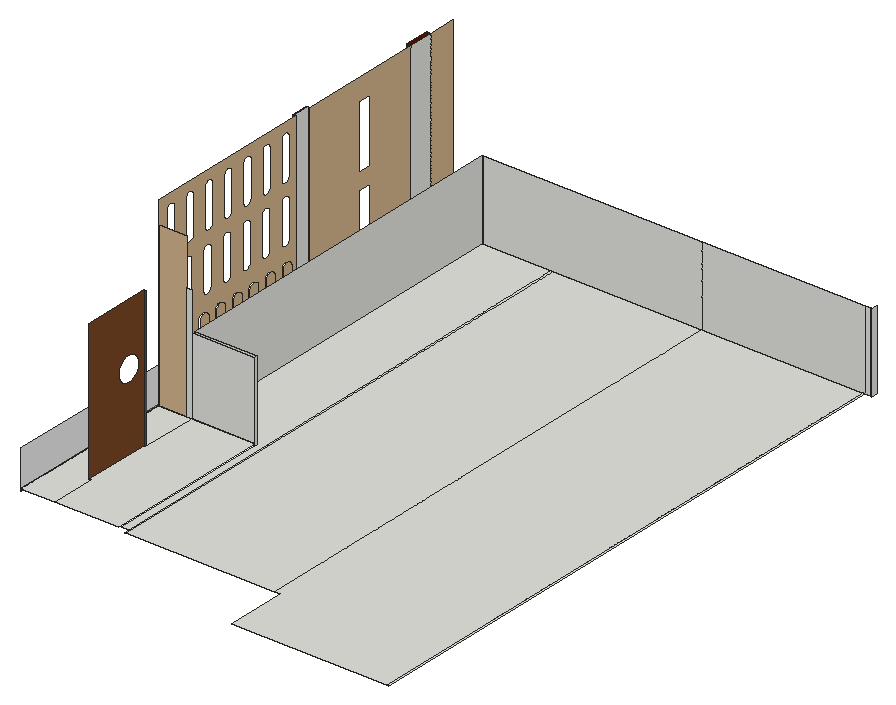
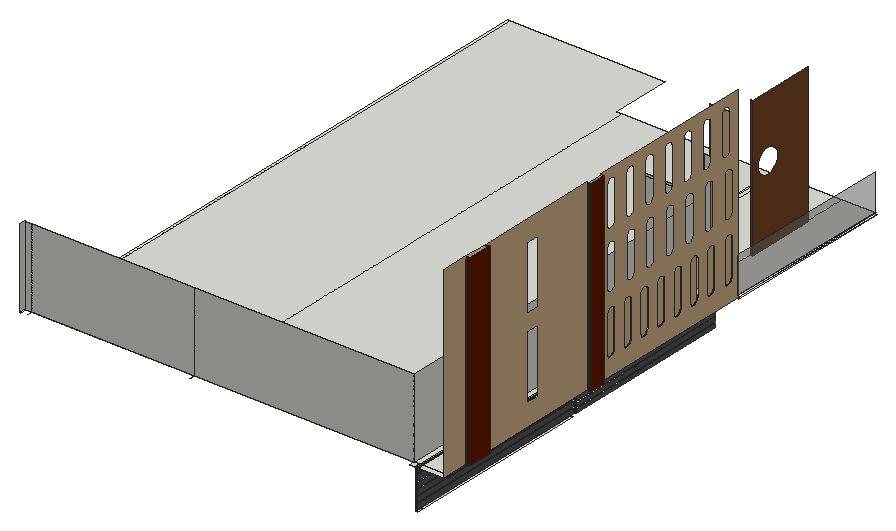
# SketchUp Ruby script. Lengths in inches.
U = 1.inch
M = Sketchup.active_model
def pt(a) = Geom::Point3d.new(a.map { |v| v * U })
def face(e, loops, mat)
  f = e.add_face(loops[0].map { |a| pt(a) })
  loops[1..].each { |l| e.add_face(l.map { |a| pt(a) }).erase! }
  f.material = f.back_material = mat if mat
  f
end
# faces: each face lists its corners as indices into pts; further lists are holes
def faces(e, pts, list, mat = nil) = list.each { |f| face(e, (f[0].is_a?(Array) ? f : [f]).map { |l| l.map { |i| pts[i] } }, mat) }
# xy, xz, yz: faces in a plane at the given z, y or x. An outline is a flat list of corners, or four numbers for a rectangle; further outlines are holes
def ring(l) = l.size == 4 ? [[l[0], l[1]], [l[2], l[1]], [l[2], l[3]], [l[0], l[3]]] : l.each_slice(2).to_a
def flat(e, list, mat, &to3) = list.each { |f| face(e, (f[0].is_a?(Array) ? f : [f]).map { |l| ring(l).map { |u, v| to3.(u, v) } }, mat) }
def xy(e, z, list, mat = nil) = flat(e, list, mat) { |x, y| [x, y, z] }
def xz(e, y, list, mat = nil) = flat(e, list, mat) { |x, z| [x, y, z] }
def yz(e, x, list, mat = nil) = flat(e, list, mat) { |y, z| [x, y, z] }
def lines(e, pts, list) = list.each { |a, b| e.add_line(pt(pts[a]), pt(pts[b])) }
# prism: a flat outline (further loops are holes) pulled along v
def prism(e, loops, v, mat = nil)
  f = face(e, loops, mat); d = Geom::Vector3d.new(v.map { |x| x * U })
  f.pushpull(f.normal.samedirection?(d) ? d.length : -d.length)
end
def box(e, o, s, mat = nil) = prism(e, [[o, [o[0] + s[0], o[1], o[2]], [o[0] + s[0], o[1] + s[1], o[2]], [o[0], o[1] + s[1], o[2]]]], [0, 0, s[2]], mat)
def at(x, y, z, deg = 0) = Geom::Transformation.translation(pt([x, y, z])) * Geom::Transformation.rotation(ORIGIN, Z_AXIS, deg.degrees)
def axes(o, x, y, z) = Geom::Transformation.new([*x, 0, *y, 0, *z, 0, *pt(o).to_a, 1])
def part(name) = M.definitions.add(name)
# library, detail: a bought-in or finely detailed component or shape, given as its bounding box
def library(name, o, s) = part(name).tap { |d| box(d.entities, o, s) }
def detail(e, o, s) = box(e.add_group.entities, o, s)
def put(e, d, t, mat = nil) = e.add_instance(d, t).tap { |i| i.material = mat if mat }
def group(e, t, mat = nil) = e.add_group.tap { |g| g.transformation = t; g.material = mat if mat }.entities
root = M.entities
M.materials.add("[0035_Tan]").color = [210, 180, 140]
M.materials.add("[Color B08]").color = [102, 25, 0]
M.materials.add("[Color M06]").color = [86, 86, 86]
M.materials.add("[Translucent Glass Gray]").color = [128, 128, 128]
M.materials["[Translucent Glass Gray]"].alpha = 0.5
M.materials.add("[Wood Veneer 01]").color = [120, 70, 37]
xy(root,120.75,[[90.83,1025.52,93.83,1311.7],[90.83,1311.7,93.83,1320.7]])
xy(root,122.27,[[90.83,755.01,93.83,1019.03]])
xy(root,123.5,[[90.83,1025.52,93.83,1320.7]])
xy(root,128.25,[[90.83,755.01,93.83,761.77],[90.83,761.77,93.83,1019.03]])
xy(root,130.625,[[90.83,1025.52,93.83,1311.7],[90.83,1311.7,93.83,1320.7]])
xy(root,130.89,[[90.83,755.01,93.83,1019.03]])
xy(root,133.375,[[90.83,1025.52,93.83,1320.7]])
xy(root,136.875,[[90.83,755.01,93.83,761.77],[90.83,761.77,93.83,1019.03]])
xy(root,139.52,[[90.83,755.01,93.83,1019.03]])
xy(root,140.5,[[90.83,1025.52,93.83,1311.7],[90.83,1311.7,93.83,1320.7]])
xy(root,143.25,[[90.83,1025.52,93.83,1320.7]])
xy(root,145.5,[[90.83,755.01,93.83,761.77],[90.83,761.77,93.83,1019.03]])
xy(root,148.14,[[90.83,755.01,93.83,1019.03]])
xy(root,150.375,[[90.83,1025.52,93.83,1311.7],[90.83,1311.7,93.83,1320.7]])
xy(root,153.125,[[90.83,1025.52,93.83,1320.7]])
xy(root,154.125,[[90.83,755.01,93.83,761.77],[90.83,761.77,93.83,1019.03]])
xy(root,156.77,[[90.83,755.01,93.83,1019.03]])
xy(root,160.25,[[90.83,1025.52,93.83,1311.7],[90.83,1311.7,93.83,1320.7]])
xy(root,162.75,[[90.83,755.01,93.83,761.77],[90.83,761.77,93.83,1019.03]])
xy(root,163,[[90.83,1025.52,93.83,1320.7]])
xy(root,165.39,[[90.83,755.01,93.83,1019.03]])
xy(root,170.125,[[90.83,1025.52,93.83,1311.7],[90.83,1311.7,93.83,1320.7]])
xy(root,171.375,[[90.83,755.01,93.83,761.77],[90.83,761.77,93.83,1019.03]])
xy(root,172.875,[[90.83,1025.52,93.83,1320.7]])
xy(root,174.02,[[90.83,755.01,93.83,1019.03]])
xy(root,180,[[446.36,406.51,446.36,499.93,437.36,499.93,437.36,1311.7,681.83,1311.7,681.83,406.51],[681.83,406.51,681.89,1311.7],[681.89,406.51,684.83,1311.7],[436.7,499.93,210.36,500.32,210.36,1311.7,436.7,1311.7],[436.7,499.93,437.36,1311.7],
  [208.04,500.32,210.36,1311.7],[49.08,501.15,49.08,761.77,51.64,761.77],[93.83,508.43,100.83,761.77],[100.83,508.43,102.83,761.77],[197.39,508.43,197.39,765.46,102.83,765.46,102.83,1311.7,208.04,1311.7,208.04,508.43],
  [90.83,755.01,93.83,761.77],[51.64,761.77,51.64,1022.51,48.64,1022.51,48.64,1047.49,51.64,1047.49,51.64,1311.7,90.83,1311.7,90.83,1025.52,87.83,1025.52,87.83,1019.03,90.83,1019.03,90.83,761.77],[93.83,761.77,93.83,1019.03,87.83,1019.03,87.83,1025.52,93.83,1025.52,93.83,1311.7,102.83,1311.7,102.83,761.77],[90.83,761.77,93.83,1019.03],[102.83,761.77,197.39,765.46],
  [102.83,761.77,197.39,765.46],[45.64,1022.51,48.64,1047.49],[90.83,1025.52,93.83,1311.7],[45.64,1240.86,51.64,1277.54],[51.64,1311.7,90.83,1320.7],
  [90.83,1311.7,93.83,1320.7],[93.83,1311.7,94.96,1320.7],[94.96,1311.7,102.83,1320.7],[693.83,1311.7,695.08,1320.7]])
xy(root,182.9375,[[49.08,502.77,49.1,502.77,51.64,761.77,49.08,761.77],[49.1,502.77,100.83,502.77,100.83,570.62,97.83,570.62,97.83,675.43,100.83,675.43,100.83,761.77,51.64,761.77],[100.83,502.77,197.39,502.77,197.39,761.77,100.83,761.77,100.83,675.43,97.83,675.43,97.83,570.62,100.83,570.62]])
xz(root,675.43,[[97.83,182.9375,100.83,394.5]],"[Wood Veneer 01]")
xz(root,755.01,[[90.83,122.27,93.83,128.25],[90.83,130.89,93.83,136.875],[90.83,139.52,93.83,145.5],[90.83,148.14,93.83,154.125],[90.83,156.77,93.83,162.75],
  [90.83,165.39,93.83,171.375],[90.83,174.02,93.83,180]])
xz(root,761.77,[[49.08,180,51.64,182.9375],[51.64,180,93.83,182.9375],[93.83,180,100.83,182.9375],[100.83,180,102.83,182.9375],[102.83,180,197.39,182.9375],
  [93.83,182.9375,100.83,358.375],[100.83,182.9375,197.39,300]])
xz(root,761.77,[[51.64,182.9375,93.83,429.125]],"[0035_Tan]")
xz(root,765.46,[[102.83,180,197.39,300]])
xz(root,1019.03,[[90.83,122.27,93.83,128.25],[90.83,130.89,93.83,136.875],[90.83,139.52,93.83,145.5],[90.83,148.14,93.83,154.125],[90.83,156.77,93.83,162.75],
  [90.83,165.39,93.83,171.375],[90.83,174.02,93.83,180]])
xz(root,1022.51,[[45.64,180,48.64,463.1875],[48.64,180,51.64,463.1875]],"[Color B08]")
xz(root,1025.52,[[90.83,123.5,93.83,130.625],[90.83,133.375,93.83,140.5],[90.83,143.25,93.83,150.375],[90.83,153.125,93.83,160.25],[90.83,163,93.83,170.125],
  [90.83,172.875,93.83,180]])
xz(root,1047.49,[[45.64,180,48.64,463.1875],[48.64,180,51.64,463.1875]],"[Color B08]")
xz(root,1240.86,[[45.64,180,51.64,463.1875]],"[Color B08]")
xz(root,1277.54,[[45.64,180,51.64,463.1875]],"[Color B08]")
xz(root,1311.7,[[102.83,180,103.71,300],[103.71,180,436.7,300],[436.7,180,684.83,300],[684.83,180,693.83,300],[693.83,180,695.08,300]])
xz(root,1320.7,[[90.83,123.5,93.83,130.625],[90.83,133.375,93.83,140.5],[90.83,143.25,93.83,150.375],[90.83,153.125,93.83,160.25],[90.83,163,93.83,170.125],
  [90.83,172.875,93.83,180]])
yz(root,45.64,[[1022.51,180,1047.49,463.1875],[1240.86,180,1277.54,463.1875]],"[Color B08]")
yz(root,48.64,[[1022.51,180,1047.49,463.1875]])
yz(root,51.64,[[1240.86,180,1277.54,463.1875]])
yz(root,51.64,[[[761.77,180,1022.51,463.1875],[1002.08,380.5625,1004.08,380.83,1005.94,381.6,1007.54,382.82,1008.77,384.42,1009.54,386.28,1009.8,388.28,1009.8,443.41,1009.2,445.06,1008.24,446.53,1006.99,447.77,1005.49,448.69,1003.83,449.27,1002.08,449.46,1000.33,449.27,998.67,448.69,997.18,447.77,995.92,446.53,994.97,445.06,994.36,443.41,994.36,388.28,994.625,386.28,995.4,384.42,996.625,382.82,998.22,381.6,1000.08,380.83],[965.71,380.5625,967.7,380.83,969.57,381.6,971.16,382.82,972.39,384.42,973.16,386.28,973.43,388.28,973.43,443.41,972.82,445.06,971.87,446.53,970.61,447.77,969.12,448.69,967.45,449.27,965.71,449.46,963.96,449.27,962.3,448.69,960.8,447.77,959.55,446.53,958.59,445.06,957.99,443.41,957.99,388.28,958.25,386.28,959.02,384.42,960.25,382.82,961.85,381.6,963.71,380.83],[929.33,380.5625,931.33,380.83,933.19,381.6,934.79,382.82,936.02,384.42,936.79,386.28,937.05,388.28,937.05,443.41,936.45,445.06,935.49,446.53,934.24,447.77,932.74,448.69,931.08,449.27,929.33,449.46,927.58,449.27,925.92,448.69,924.43,447.77,923.17,446.53,922.22,445.06,921.61,443.41,921.61,388.28,921.875,386.28,922.65,384.42,923.875,382.82,925.47,381.6,927.33,380.83],[892.96,380.5625,894.95,380.83,896.82,381.6,898.41,382.82,899.64,384.42,900.41,386.28,900.68,388.28,900.68,443.41,900.07,445.06,899.12,446.53,897.86,447.77,896.37,448.69,894.7,449.27,892.96,449.46,891.21,449.27,889.55,448.69,888.05,447.77,886.8,446.53,885.84,445.06,885.24,443.41,885.24,388.28,885.5,386.28,886.27,384.42,887.5,382.82,889.1,381.6,890.96,380.83],[856.58,380.5625,858.58,380.83,860.44,381.6,862.04,382.82,863.27,384.42,864.04,386.28,864.3,388.28,864.3,443.41,863.7,445.06,862.74,446.53,861.49,447.77,859.99,448.69,858.33,449.27,856.58,449.46,854.83,449.27,853.17,448.69,851.68,447.77,850.42,446.53,849.47,445.06,848.86,443.41,848.86,388.28,849.125,386.28,849.9,384.42,851.125,382.82,852.72,381.6,854.58,380.83],[820.21,380.5625,822.2,380.83,824.07,381.6,825.66,382.82,826.89,384.42,827.66,386.28,827.93,388.28,827.93,443.41,827.32,445.06,826.37,446.53,825.11,447.77,823.62,448.69,821.95,449.27,820.21,449.46,818.46,449.27,816.8,448.69,815.3,447.77,814.05,446.53,813.09,445.06,812.49,443.41,812.49,388.28,812.75,386.28,813.52,384.42,814.75,382.82,816.35,381.6,818.21,380.83],[783.83,380.5625,785.83,380.83,787.69,381.6,789.29,382.82,790.52,384.42,791.29,386.28,791.55,388.28,791.55,443.41,790.95,445.06,789.99,446.53,788.74,447.77,787.24,448.69,785.58,449.27,783.83,449.46,782.08,449.27,780.42,448.69,778.93,447.77,777.67,446.53,776.72,445.06,776.11,443.41,776.11,388.28,776.375,386.28,777.15,384.42,778.375,382.82,779.97,381.6,781.83,380.83],[1002.08,294.25,1004.08,294.51,1005.94,295.28,1007.54,296.51,1008.77,298.11,1009.54,299.97,1009.8,301.97,1009.8,357.09,1009.2,358.74,1008.24,360.22,1006.99,361.45,1005.49,362.38,1003.83,362.95,1002.08,363.15,1000.33,362.95,998.67,362.38,997.18,361.45,995.92,360.22,994.97,358.74,994.36,357.09,994.36,301.97,994.625,299.97,995.4,298.11,996.625,296.51,998.22,295.28,1000.08,294.51],[964.89,294.25,966.89,294.51,968.75,295.28,970.35,296.51,971.58,298.11,972.35,299.97,972.61,301.97,972.61,357.09,972.01,358.74,971.05,360.22,969.8,361.45,968.3,362.38,966.64,362.95,964.89,363.15,963.15,362.95,961.48,362.38,959.99,361.45,958.73,360.22,957.78,358.74,957.18,357.09,957.18,301.97,957.4375,299.97,958.21,298.11,959.4375,296.51,961.04,295.28,962.9,294.51],[927.71,294.25,929.7,294.51,931.57,295.28,933.16,296.51,934.39,298.11,935.16,299.97,935.43,301.97,935.43,357.09,934.82,358.74,933.87,360.22,932.61,361.45,931.12,362.38,929.45,362.95,927.71,363.15,925.96,362.95,924.3,362.38,922.8,361.45,921.55,360.22,920.59,358.74,919.99,357.09,919.99,301.97,920.25,299.97,921.02,298.11,922.25,296.51,923.85,295.28,925.71,294.51],[890.52,294.25,892.52,294.51,894.38,295.28,895.98,296.51,897.2,298.11,897.98,299.97,898.24,301.97,898.24,357.09,897.63,358.74,896.68,360.22,895.42,361.45,893.93,362.38,892.27,362.95,890.52,363.15,888.77,362.95,887.11,362.38,885.61,361.45,884.36,360.22,883.41,358.74,882.8,357.09,882.8,301.97,883.0625,299.97,883.83,298.11,885.0625,296.51,886.66,295.28,888.52,294.51],[853.33,294.25,855.33,294.51,857.19,295.28,858.79,296.51,860.02,298.11,860.79,299.97,861.05,301.97,861.05,357.09,860.45,358.74,859.49,360.22,858.24,361.45,856.74,362.38,855.08,362.95,853.33,363.15,851.58,362.95,849.92,362.38,848.43,361.45,847.17,360.22,846.22,358.74,845.61,357.09,845.61,301.97,845.875,299.97,846.65,298.11,847.875,296.51,849.47,295.28,851.33,294.51],[816.14,294.25,818.14,294.51,820,295.28,821.6,296.51,822.83,298.11,823.6,299.97,823.86,301.97,823.86,357.09,823.26,358.74,822.3,360.22,821.05,361.45,819.55,362.38,817.89,362.95,816.14,363.15,814.4,362.95,812.73,362.38,811.24,361.45,809.98,360.22,809.03,358.74,808.43,357.09,808.43,301.97,808.6875,299.97,809.46,298.11,810.6875,296.51,812.29,295.28,814.15,294.51],[778.96,294.25,780.95,294.51,782.82,295.28,784.41,296.51,785.64,298.11,786.41,299.97,786.68,301.97,786.68,357.09,786.07,358.74,785.12,360.22,783.86,361.45,782.37,362.38,780.7,362.95,778.96,363.15,777.21,362.95,775.55,362.38,774.05,361.45,772.8,360.22,771.84,358.74,771.24,357.09,771.24,301.97,771.5,299.97,772.27,298.11,773.5,296.51,775.1,295.28,776.96,294.51],[1002.08,204.75,1004.08,205.01,1005.94,205.78,1007.54,207.01,1008.77,208.61,1009.54,210.47,1009.8,212.47,1009.8,267.59,1009.2,269.24,1008.24,270.72,1006.99,271.95,1005.49,272.88,1003.83,273.45,1002.08,273.65,1000.33,273.45,998.67,272.88,997.18,271.95,995.92,270.72,994.97,269.24,994.36,267.59,994.36,212.47,994.625,210.47,995.4,208.61,996.625,207.01,998.22,205.78,1000.08,205.01],[970.46,204.75,972.45,205.01,974.32,205.78,975.91,207.01,977.14,208.61,977.91,210.47,978.18,212.47,978.18,267.59,977.57,269.24,976.62,270.72,975.36,271.95,973.87,272.88,972.2,273.45,970.46,273.65,968.71,273.45,967.05,272.88,965.55,271.95,964.3,270.72,963.34,269.24,962.74,267.59,962.74,212.47,963,210.47,963.77,208.61,965,207.01,966.6,205.78,968.46,205.01],[938.83,204.75,940.83,205.01,942.69,205.78,944.29,207.01,945.52,208.61,946.29,210.47,946.55,212.47,946.55,267.59,945.95,269.24,944.99,270.72,943.74,271.95,942.24,272.88,940.58,273.45,938.83,273.65,937.08,273.45,935.42,272.88,933.93,271.95,932.67,270.72,931.72,269.24,931.11,267.59,931.11,212.47,931.375,210.47,932.15,208.61,933.375,207.01,934.97,205.78,936.83,205.01],[907.21,204.75,909.2,205.01,911.07,205.78,912.66,207.01,913.89,208.61,914.66,210.47,914.93,212.47,914.93,267.59,914.32,269.24,913.37,270.72,912.11,271.95,910.62,272.88,908.95,273.45,907.21,273.65,905.46,273.45,903.8,272.88,902.3,271.95,901.05,270.72,900.09,269.24,899.49,267.59,899.49,212.47,899.75,210.47,900.52,208.61,901.75,207.01,903.35,205.78,905.21,205.01],[875.58,204.75,877.58,205.01,879.44,205.78,881.04,207.01,882.27,208.61,883.04,210.47,883.3,212.47,883.3,267.59,882.7,269.24,881.74,270.72,880.49,271.95,878.99,272.88,877.33,273.45,875.58,273.65,873.83,273.45,872.17,272.88,870.68,271.95,869.42,270.72,868.47,269.24,867.86,267.59,867.86,212.47,868.125,210.47,868.9,208.61,870.125,207.01,871.72,205.78,873.58,205.01],[843.96,204.75,845.95,205.01,847.82,205.78,849.41,207.01,850.64,208.61,851.41,210.47,851.68,212.47,851.68,267.59,851.07,269.24,850.12,270.72,848.86,271.95,847.37,272.88,845.7,273.45,843.96,273.65,842.21,273.45,840.55,272.88,839.05,271.95,837.8,270.72,836.84,269.24,836.24,267.59,836.24,212.47,836.5,210.47,837.27,208.61,838.5,207.01,840.1,205.78,841.96,205.01],[812.33,204.75,814.33,205.01,816.19,205.78,817.79,207.01,819.02,208.61,819.79,210.47,820.05,212.47,820.05,267.59,819.45,269.24,818.49,270.72,817.24,271.95,815.74,272.88,814.08,273.45,812.33,273.65,810.58,273.45,808.92,272.88,807.43,271.95,806.17,270.72,805.22,269.24,804.61,267.59,804.61,212.47,804.875,210.47,805.65,208.61,806.875,207.01,808.47,205.78,810.33,205.01],[778.46,204.75,780.45,205.01,782.32,205.78,783.91,207.01,785.14,208.61,785.91,210.47,786.18,212.47,786.18,267.59,785.57,269.24,784.62,270.72,783.36,271.95,781.87,272.88,780.2,273.45,778.46,273.65,776.71,273.45,775.05,272.88,773.55,271.95,772.3,270.72,771.34,269.24,770.74,267.59,770.74,212.47,771,210.47,771.77,208.61,773,207.01,774.6,205.78,776.46,205.01]],[[1047.49,180,1240.86,463.1875],[1140.89,334,1161.64,430.9375],[1140.89,212.375,1161.64,309.3125]],[1277.54,180,1320.7,463.1875]],"[0035_Tan]")
yz(root,54.64,[[778.46,204.75,776.46,205.01,774.6,205.78,773,207.01,771.77,208.61,771,210.47,770.74,212.47,770.74,267.59,771.34,269.24,772.3,270.72,773.55,271.95,775.05,272.88,776.71,273.45,778.46,273.65,780.2,273.45,781.87,272.88,783.36,271.95,784.62,270.72,785.57,269.24,786.18,267.59,786.18,212.47,785.91,210.47,785.14,208.61,783.91,207.01,782.32,205.78,780.45,205.01],[875.58,204.75,873.58,205.01,871.72,205.78,870.125,207.01,868.9,208.61,868.125,210.47,867.86,212.47,867.86,267.59,868.47,269.24,869.42,270.72,870.68,271.95,872.17,272.88,873.83,273.45,875.58,273.65,877.33,273.45,878.99,272.88,880.49,271.95,881.74,270.72,882.7,269.24,883.3,267.59,883.3,212.47,883.04,210.47,882.27,208.61,881.04,207.01,879.44,205.78,877.58,205.01],[907.21,204.75,905.21,205.01,903.35,205.78,901.75,207.01,900.52,208.61,899.75,210.47,899.49,212.47,899.49,267.59,900.09,269.24,901.05,270.72,902.3,271.95,903.8,272.88,905.46,273.45,907.21,273.65,908.95,273.45,910.62,272.88,912.11,271.95,913.37,270.72,914.32,269.24,914.93,267.59,914.93,212.47,914.66,210.47,913.89,208.61,912.66,207.01,911.07,205.78,909.2,205.01],[938.83,204.75,936.83,205.01,934.97,205.78,933.375,207.01,932.15,208.61,931.375,210.47,931.11,212.47,931.11,267.59,931.72,269.24,932.67,270.72,933.93,271.95,935.42,272.88,937.08,273.45,938.83,273.65,940.58,273.45,942.24,272.88,943.74,271.95,944.99,270.72,945.95,269.24,946.55,267.59,946.55,212.47,946.29,210.47,945.52,208.61,944.29,207.01,942.69,205.78,940.83,205.01],[970.46,204.75,968.46,205.01,966.6,205.78,965,207.01,963.77,208.61,963,210.47,962.74,212.47,962.74,267.59,963.34,269.24,964.3,270.72,965.55,271.95,967.05,272.88,968.71,273.45,970.46,273.65,972.2,273.45,973.87,272.88,975.36,271.95,976.62,270.72,977.57,269.24,978.18,267.59,978.18,212.47,977.91,210.47,977.14,208.61,975.91,207.01,974.32,205.78,972.45,205.01],
  [1002.08,204.75,1000.08,205.01,998.22,205.78,996.625,207.01,995.4,208.61,994.625,210.47,994.36,212.47,994.36,267.59,994.97,269.24,995.92,270.72,997.18,271.95,998.67,272.88,1000.33,273.45,1002.08,273.65,1003.83,273.45,1005.49,272.88,1006.99,271.95,1008.24,270.72,1009.2,269.24,1009.8,267.59,1009.8,212.47,1009.54,210.47,1008.77,208.61,1007.54,207.01,1005.94,205.78,1004.08,205.01]],"[0035_Tan]")
yz(root,55.14,[[812.33,204.75,810.33,205.01,808.47,205.78,806.875,207.01,805.65,208.61,804.875,210.47,804.61,212.47,804.61,267.59,805.22,269.24,806.17,270.72,807.43,271.95,808.92,272.88,810.58,273.45,812.33,273.65,814.08,273.45,815.74,272.88,817.24,271.95,818.49,270.72,819.45,269.24,820.05,267.59,820.05,212.47,819.79,210.47,819.02,208.61,817.79,207.01,816.19,205.78,814.33,205.01],[843.96,204.75,841.96,205.01,840.1,205.78,838.5,207.01,837.27,208.61,836.5,210.47,836.24,212.47,836.24,267.59,836.84,269.24,837.8,270.72,839.05,271.95,840.55,272.88,842.21,273.45,843.96,273.65,845.7,273.45,847.37,272.88,848.86,271.95,850.12,270.72,851.07,269.24,851.68,267.59,851.68,212.47,851.41,210.47,850.64,208.61,849.41,207.01,847.82,205.78,845.95,205.01]],"[0035_Tan]")
yz(root,90.83,[[755.01,122.27,1019.03,128.25],[1025.52,123.5,1320.7,130.625],[755.01,130.89,1019.03,136.875],[1025.52,133.375,1320.7,140.5],[755.01,139.52,1019.03,145.5],
  [1025.52,143.25,1320.7,150.375],[755.01,148.14,1019.03,154.125],[1025.52,153.125,1320.7,160.25],[755.01,156.77,1019.03,162.75],[1025.52,163,1320.7,170.125],
  [755.01,165.39,1019.03,171.375],[1025.52,172.875,1320.7,180],[755.01,174.02,1019.03,180]],"[Color M06]")
yz(root,93.83,[[1025.52,120.75,1320.7,123.5],[755.01,122.27,1019.03,128.25],[1025.52,123.5,1320.7,130.625],[1025.52,130.625,1320.7,133.375],[755.01,130.89,1019.03,136.875],
  [1025.52,133.375,1320.7,140.5],[755.01,136.875,1019.03,139.52],[755.01,139.52,1019.03,145.5],[1025.52,140.5,1320.7,143.25],[1025.52,143.25,1320.7,150.375],
  [755.01,145.5,1019.03,148.14],[755.01,148.14,1019.03,154.125],[1025.52,150.375,1320.7,153.125],[1025.52,153.125,1320.7,160.25],[755.01,154.125,1019.03,156.77],
  [755.01,156.77,1019.03,162.75],[1025.52,160.25,1320.7,163],[755.01,162.75,1019.03,165.39],[1025.52,163,1320.7,170.125],[755.01,165.39,1019.03,171.375],
  [1025.52,170.125,1320.7,172.875],[755.01,171.375,1019.03,174.02],[1025.52,172.875,1320.7,180],[755.01,174.02,1019.03,180]])
yz(root,93.83,[[755.01,128.25,1019.03,130.89]],"[Color M06]")
yz(root,97.83,[[[570.62,182.9375,675.43,394.5],[646.43,281.17,651.33,281.82,655.9,283.71,659.82,286.72,662.83,290.64,664.72,295.21,665.36,300.11,664.72,305.01,662.83,309.58,659.82,313.5,655.9,316.51,651.33,318.4,646.43,319.05,641.53,318.4,636.96,316.51,633.04,313.5,630.03,309.58,628.13,305.01,627.49,300.11,628.13,295.21,630.03,290.64,633.04,286.72,636.96,283.71,641.53,281.82]]],"[Wood Veneer 01]")
yz(root,102.83,[[765.46,180,1311.7,300]])
yz(root,197.39,[[761.77,180,765.46,300]])
yz(root,695.08,[[1311.7,180,1320.7,300]])
p = [[51.64,761.77,182.9375],[49.1,502.77,182.9375],[49.1,502.77,238.85],[51.64,761.77,238.85],[51.64,778.46,204.75],[51.64,776.46,205.01],
  [54.64,776.46,205.01],[54.64,778.46,204.75],[51.64,780.45,205.01],[54.64,780.45,205.01],[51.64,812.33,204.75],[51.64,810.33,205.01],
  [55.14,810.33,205.01],[55.14,812.33,204.75],[51.64,814.33,205.01],[55.14,814.33,205.01],[51.64,843.96,204.75],[51.64,841.96,205.01],
  [55.14,841.96,205.01],[55.14,843.96,204.75],[51.64,845.95,205.01],[55.14,845.95,205.01],[51.64,875.58,204.75],[51.64,873.58,205.01],
  [54.64,873.58,205.01],[54.64,875.58,204.75],[51.64,877.58,205.01],[54.64,877.58,205.01],[51.64,907.21,204.75],[51.64,905.21,205.01],
  [54.64,905.21,205.01],[54.64,907.21,204.75],[51.64,909.2,205.01],[54.64,909.2,205.01],[51.64,938.83,204.75],[51.64,936.83,205.01],
  [54.64,936.83,205.01],[54.64,938.83,204.75],[51.64,940.83,205.01],[54.64,940.83,205.01],[51.64,970.46,204.75],[51.64,968.46,205.01],
  [54.64,968.46,205.01],[54.64,970.46,204.75],[51.64,972.45,205.01],[54.64,972.45,205.01],[51.64,1002.08,204.75],[51.64,1000.08,205.01],
  [54.64,1000.08,205.01],[54.64,1002.08,204.75],[51.64,1004.08,205.01],[54.64,1004.08,205.01],[51.64,774.6,205.78],[54.64,774.6,205.78],
  [51.64,782.32,205.78],[54.64,782.32,205.78],[51.64,808.47,205.78],[55.14,808.47,205.78],[51.64,816.19,205.78],[55.14,816.19,205.78],
  [51.64,840.1,205.78],[55.14,840.1,205.78],[51.64,847.82,205.78],[55.14,847.82,205.78],[51.64,871.72,205.78],[54.64,871.72,205.78],
  [51.64,879.44,205.78],[54.64,879.44,205.78],[51.64,903.35,205.78],[54.64,903.35,205.78],[51.64,911.07,205.78],[54.64,911.07,205.78],
  [51.64,934.97,205.78],[54.64,934.97,205.78],[51.64,942.69,205.78],[54.64,942.69,205.78],[51.64,966.6,205.78],[54.64,966.6,205.78],
  [51.64,974.32,205.78],[54.64,974.32,205.78],[51.64,998.22,205.78],[54.64,998.22,205.78],[51.64,1005.94,205.78],[54.64,1005.94,205.78],
  [51.64,773,207.01],[54.64,773,207.01],[51.64,783.91,207.01],[54.64,783.91,207.01],[51.64,806.875,207.01],[55.14,806.875,207.01],
  [51.64,817.79,207.01],[55.14,817.79,207.01],[51.64,838.5,207.01],[55.14,838.5,207.01],[51.64,849.41,207.01],[55.14,849.41,207.01],
  [51.64,870.125,207.01],[54.64,870.125,207.01],[51.64,881.04,207.01],[54.64,881.04,207.01],[51.64,901.75,207.01],[54.64,901.75,207.01],
  [51.64,912.66,207.01],[54.64,912.66,207.01],[51.64,933.375,207.01],[54.64,933.375,207.01],[51.64,944.29,207.01],[54.64,944.29,207.01],
  [51.64,965,207.01],[54.64,965,207.01],[51.64,975.91,207.01],[54.64,975.91,207.01],[51.64,996.625,207.01],[54.64,996.625,207.01],
  [51.64,1007.54,207.01],[54.64,1007.54,207.01],[51.64,771.77,208.61],[54.64,771.77,208.61],[51.64,785.14,208.61],[54.64,785.14,208.61],
  [51.64,805.65,208.61],[55.14,805.65,208.61],[51.64,819.02,208.61],[55.14,819.02,208.61],[51.64,837.27,208.61],[55.14,837.27,208.61],
  [51.64,850.64,208.61],[55.14,850.64,208.61],[51.64,868.9,208.61],[54.64,868.9,208.61],[51.64,882.27,208.61],[54.64,882.27,208.61],
  [51.64,900.52,208.61],[54.64,900.52,208.61],[51.64,913.89,208.61],[54.64,913.89,208.61],[51.64,932.15,208.61],[54.64,932.15,208.61],
  [51.64,945.52,208.61],[54.64,945.52,208.61],[51.64,963.77,208.61],[54.64,963.77,208.61],[51.64,977.14,208.61],[54.64,977.14,208.61],
  [51.64,995.4,208.61],[54.64,995.4,208.61],[51.64,1008.77,208.61],[54.64,1008.77,208.61],[51.64,771,210.47],[54.64,771,210.47],
  [51.64,785.91,210.47],[54.64,785.91,210.47],[51.64,804.875,210.47],[55.14,804.875,210.47],[51.64,819.79,210.47],[55.14,819.79,210.47],
  [51.64,836.5,210.47],[55.14,836.5,210.47],[51.64,851.41,210.47],[55.14,851.41,210.47],[51.64,868.125,210.47],[54.64,868.125,210.47],
  [51.64,883.04,210.47],[54.64,883.04,210.47],[51.64,899.75,210.47],[54.64,899.75,210.47],[51.64,914.66,210.47],[54.64,914.66,210.47],
  [51.64,931.375,210.47],[54.64,931.375,210.47],[51.64,946.29,210.47],[54.64,946.29,210.47],[51.64,963,210.47],[54.64,963,210.47],
  [51.64,977.91,210.47],[54.64,977.91,210.47],[51.64,994.625,210.47],[54.64,994.625,210.47],[51.64,1009.54,210.47],[54.64,1009.54,210.47],
  [684.83,1311.7,180],[684.83,1320.7,180],[102.83,761.77,165],[93.83,761.77,165],[437.36,1311.7,180],[437.36,1320.7,180]]
faces(root,p,[[0,1,2,3]],"[Translucent Glass Gray]")
faces(root,p,[[4,5,6,7],[8,4,7,9],[10,11,12,13],[14,10,13,15],[16,17,18,19],[20,16,19,21],[22,23,24,25],[26,22,25,27],
  [28,29,30,31],[32,28,31,33],[34,35,36,37],[38,34,37,39],[40,41,42,43],[44,40,43,45],[46,47,48,49],[50,46,49,51],
  [5,52,53,6],[54,8,9,55],[11,56,57,12],[58,14,15,59],[17,60,61,18],[62,20,21,63],[23,64,65,24],[66,26,27,67],
  [29,68,69,30],[70,32,33,71],[35,72,73,36],[74,38,39,75],[41,76,77,42],[78,44,45,79],[47,80,81,48],[82,50,51,83],
  [52,84,85,53],[86,54,55,87],[56,88,89,57],[90,58,59,91],[60,92,93,61],[94,62,63,95],[64,96,97,65],[98,66,67,99],
  [68,100,101,69],[102,70,71,103],[72,104,105,73],[106,74,75,107],[76,108,109,77],[110,78,79,111],[80,112,113,81],[114,82,83,115],
  [84,116,117,85],[118,86,87,119],[88,120,121,89],[122,90,91,123],[92,124,125,93],[126,94,95,127],[96,128,129,97],[130,98,99,131],
  [100,132,133,101],[134,102,103,135],[104,136,137,105],[138,106,107,139],[108,140,141,109],[142,110,111,143],[112,144,145,113],[146,114,115,147],
  [116,148,149,117],[150,118,119,151],[120,152,153,121],[154,122,123,155],[124,156,157,125],[158,126,127,159],[128,160,161,129],[162,130,131,163],
  [132,164,165,133],[166,134,135,167],[136,168,169,137],[170,138,139,171],[140,172,173,141],[174,142,143,175],[144,176,177,145],[178,146,147,179]])
lines(root,p,[[180,181],[182,183],[184,185]])
